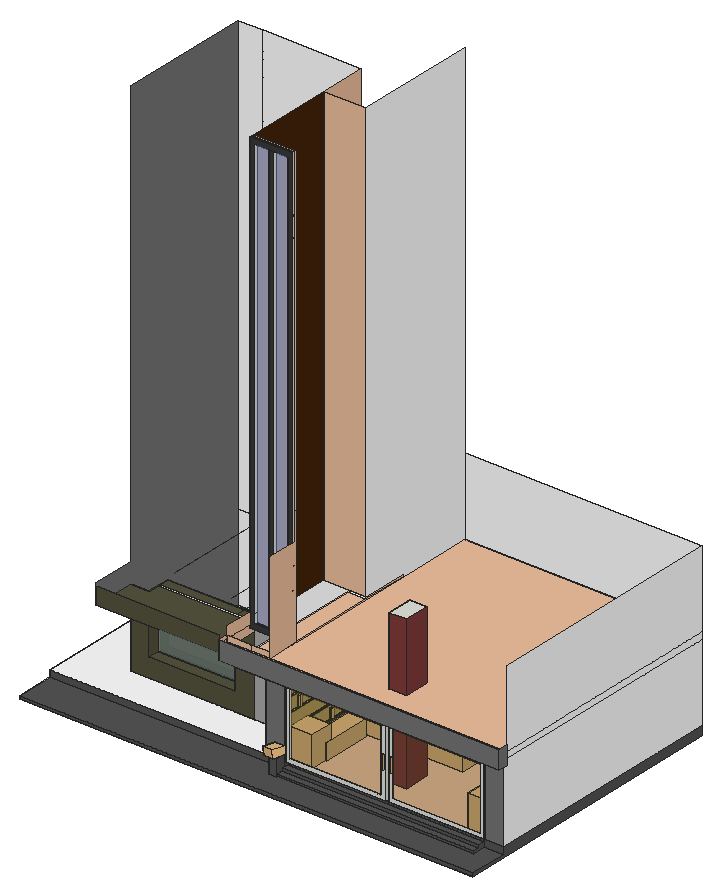
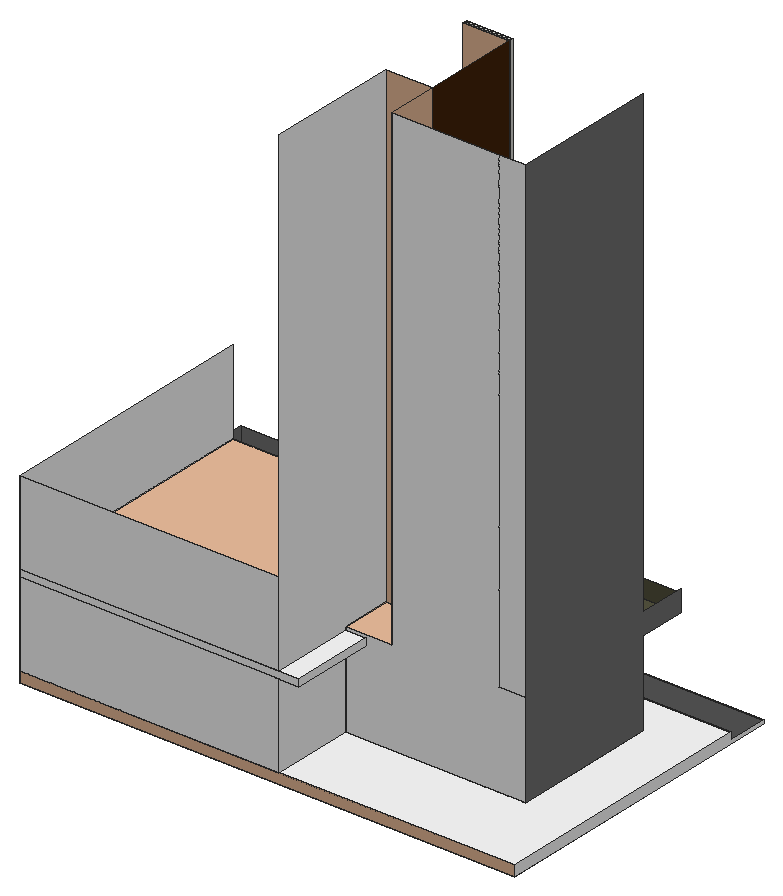
# SketchUp Ruby script. Lengths in inches.
U = 1.inch
M = Sketchup.active_model
def pt(a) = Geom::Point3d.new(a.map { |v| v * U })
def face(e, loops, mat)
  f = e.add_face(loops[0].map { |a| pt(a) })
  loops[1..].each { |l| e.add_face(l.map { |a| pt(a) }).erase! }
  f.material = f.back_material = mat if mat
  f
end
# faces: each face lists its corners as indices into pts; further lists are holes
def faces(e, pts, list, mat = nil) = list.each { |f| face(e, (f[0].is_a?(Array) ? f : [f]).map { |l| l.map { |i| pts[i] } }, mat) }
# xy, xz, yz: faces in a plane at the given z, y or x. An outline is a flat list of corners, or four numbers for a rectangle; further outlines are holes
def ring(l) = l.size == 4 ? [[l[0], l[1]], [l[2], l[1]], [l[2], l[3]], [l[0], l[3]]] : l.each_slice(2).to_a
def flat(e, list, mat, &to3) = list.each { |f| face(e, (f[0].is_a?(Array) ? f : [f]).map { |l| ring(l).map { |u, v| to3.(u, v) } }, mat) }
def xy(e, z, list, mat = nil) = flat(e, list, mat) { |x, y| [x, y, z] }
def xz(e, y, list, mat = nil) = flat(e, list, mat) { |x, z| [x, y, z] }
def yz(e, x, list, mat = nil) = flat(e, list, mat) { |y, z| [x, y, z] }
def lines(e, pts, list) = list.each { |a, b| e.add_line(pt(pts[a]), pt(pts[b])) }
# prism: a flat outline (further loops are holes) pulled along v
def prism(e, loops, v, mat = nil)
  f = face(e, loops, mat); d = Geom::Vector3d.new(v.map { |x| x * U })
  f.pushpull(f.normal.samedirection?(d) ? d.length : -d.length)
end
def box(e, o, s, mat = nil) = prism(e, [[o, [o[0] + s[0], o[1], o[2]], [o[0] + s[0], o[1] + s[1], o[2]], [o[0], o[1] + s[1], o[2]]]], [0, 0, s[2]], mat)
def at(x, y, z, deg = 0) = Geom::Transformation.translation(pt([x, y, z])) * Geom::Transformation.rotation(ORIGIN, Z_AXIS, deg.degrees)
def axes(o, x, y, z) = Geom::Transformation.new([*x, 0, *y, 0, *z, 0, *pt(o).to_a, 1])
def part(name) = M.definitions.add(name)
# library, detail: a bought-in or finely detailed component or shape, given as its bounding box
def library(name, o, s) = part(name).tap { |d| box(d.entities, o, s) }
def detail(e, o, s) = box(e.add_group.entities, o, s)
def put(e, d, t, mat = nil) = e.add_instance(d, t).tap { |i| i.material = mat if mat }
def group(e, t, mat = nil) = e.add_group.tap { |g| g.transformation = t; g.material = mat if mat }.entities
root = M.entities
M.materials.add("Generic").color = [68, 36, 11]
M.materials.add("Generic\#1").color = [84, 84, 84]
M.materials.add("Generic\#11").color = [129, 59, 59]
M.materials.add("Generic\#13").color = [239, 192, 158]
M.materials.add("Generic\#2").color = [84, 83, 62]
M.materials.add("Generic\#3").color = [117, 117, 117]
M.materials.add("Material__2").color = [190, 136, 85]
M.materials.add("Material__3").color = [51, 42, 44]
M.materials.add("Material__4").color = [119, 136, 107]
M.materials.add("[Color M00]").color = [255, 255, 255]
M.materials.add("[Color M03]").color = [170, 170, 170]
M.materials.add("[Color M07]").color = [58, 58, 58]
M.materials.add("[Mirror 02]").color = [230, 230, 157]
M.materials.add("[Translucent Glass Blue]").color = [100, 149, 237]
M.materials["[Translucent Glass Blue]"].alpha = 0.5
M.materials.add("[Translucent Glass Corrugated]").color = [177, 158, 60]
M.materials["[Translucent Glass Corrugated]"].alpha = 0.56
M.materials.add("[Translucent Glass Corrugated]1").color = [106, 119, 109]
M.materials["[Translucent Glass Corrugated]1"].alpha = 0.8
M.materials.add("[Translucent Glass Dark Green]").color = [86, 83, 28]
M.materials["[Translucent Glass Dark Green]"].alpha = 0.11
c1 = library("Plant+2 (1)",[-9.13,-9.52,0],[51.76,51.77,66.88])
c2 = library("cafe+table",[12.29,13.08,0],[75.61,73.69,46.46])
c3 = library("Group\#1",[0,0,0],[33.82,92.24,30.24])
c4 = part("Group\#7")
detail(c4.entities,[0,0,0],[1.625,2.25,24.9375])
c5 = library("\#2",[-119.83,-119.83,113.8],[239.66,239.66,17.4])
c6 = library("\#4",[-204.92,-212.35,-236.71],[424.28,257.5,472.53])
c7 = part("\#3")
put(c7.entities,c6,axes([-0.37,309.72,0],[1.36765,0,0],[0,1.36765,0],[0,0,1.36765]),"Material__4")
c8 = library("\#1",[-174.07,-174.07,0],[348.14,348.14,140])
c9 = part("9")
put(c9.entities,c5,at(-19.94,-24.66,0),"Material__3")
put(c9.entities,c7,axes([17.67,-32.6,40.29],[0.29694,0.9549,0],[-0.21403,0.06656,0.97456],[0.9306,-0.28939,0.22414]))
put(c9.entities,c8,at(-19.94,-24.66,0),"Material__2")
c10 = library("Wall Lamp 298 005",[-4.37,-9,-20.45],[8.74,9.125,40.9])
c11 = library("Untitled (6)",[-101.41,0,-4.6],[35.6,35.6,49.16])
c12 = library("Tlon Light 450 Ceiling 152 006",[-8.86,-8.86,-3.78],[17.72,17.72,3.56])
xy(root,-17.875,[[0,0,0,534.3125,848,534.3125,848,0,770.53,0,770.53,62.875,477.72,62.875,477.72,0],[477.72,0,770.53,62.875]],"Generic\#13")
xy(root,-12.4375,[[0,0,848,0,848,70.375,812,70.375,812,46.5,444.05,46.5,444.05,44.57,430.61,44.57,430.61,61.26,444.05,61.26,444.05,70.375,0,70.375]],"Generic\#1")
xy(root,-7.625,[[444.05,46.5,812,56.875]],"Generic\#1")
xy(root,-3.1875,[[444.05,56.875,812,70.375]],"Generic\#1")
xy(root,0,[[596.32,118.1875,628.39,166.25]])
xy(root,0,[[404,70.375,440,70.375,440,515.9375,812,515.9375,812,70.375,848,70.375,848,534.3125,404,534.3125],[440,70.375,442,78.3125],[442,70.375,810,514.9375],[810,70.375,812,78.3125],[440,78.3125,442,514.9375],
  [810,78.3125,812,514.9375],[94.0625,140.75,404,304.75],[94.0625,304.75,404,391.6875],[440,514.9375,812,515.9375],[440,514.9375,812,515.9375]],"Generic\#13")
xy(root,0,[[0,70.375,404,70.375,404,140.75,94.0625,140.75,94.0625,391.6875,404,391.6875,404,534.3125,0,534.3125]],"[Color M00]")
xy(root,17.3125,[[430.61,44.57,444.05,61.26]],"Generic\#1")
xy(root,23.6875,[[440,78.3125,442,514.9375],[810,78.3125,812,514.9375],[440,514.9375,812,515.9375]],"Generic\#13")
xy(root,26.6875,[[440,78.3125,442,514.9375],[810,78.3125,812,514.9375],[440,514.9375,812,515.9375]],"Generic\#13")
xy(root,35.01,[[129.07,140.75,289.24,184.8125]],"Generic\#2")
xy(root,50.375,[[440,78.3125,442,514.9375],[810,78.3125,812,514.9375],[440,514.9375,812,515.9375]],"Generic\#13")
xy(root,53.375,[[440,78.3125,442,514.9375],[810,78.3125,812,514.9375],[440,514.9375,812,515.9375]],"Generic\#13")
xy(root,77.0625,[[440,78.3125,442,514.9375],[810,78.3125,812,514.9375],[440,514.9375,812,515.9375]],"Generic\#13")
xy(root,80.0625,[[440,78.3125,442,514.9375],[810,78.3125,812,514.9375],[440,514.9375,812,515.9375]],"Generic\#13")
xy(root,103.75,[[440,78.3125,442,514.9375],[810,78.3125,812,514.9375],[440,514.9375,812,515.9375]],"Generic\#13")
xy(root,106.75,[[440,78.3125,442,514.9375],[810,78.3125,812,514.9375],[440,514.9375,812,515.9375]],"Generic\#13")
xy(root,133.4375,[[404,70.375,440,78.3125],[440,70.375,810,78.3125],[810,70.375,812,78.3125],[812,70.375,848,78.3125],[440,78.3125,442,514.9375],
  [442,78.3125,810,514.9375],[810,78.3125,812,514.9375],[440,514.9375,812,515.9375]],"Generic\#13")
xy(root,133.4375,[[324.25,60.4375,848,70.375],[324.25,70.375,404,78.3125]],"Generic\#3")
xy(root,144,[[369.1875,78.3125,404,534.3125],[404,78.3125,848,534.3125]],"Generic\#13")
xy(root,145.5625,[[94.0625,60.4375,94.0625,140.75,129.07,140.75,129.07,184.8125,289.24,184.8125,289.24,140.75,324.25,140.75,324.25,60.4375]],"Generic\#2")
xy(root,156.625,[[369.1875,78.3125,404,140.75],[404,78.3125,848,534.3125],[369.1875,140.75,404,304.75]],"Generic\#13")
xy(root,156.625,[[369.1875,304.75,404,534.3125]],"[Color M00]")
xy(root,161.19,[[324.25,304.75,404,391.6875]],"Generic\#13")
xy(root,284,[[596.32,118.1875,628.39,166.25]])
xz(root,0,[[0,-17.875,848,-12.4375]],"Generic\#1")
xz(root,44.57,[[430.61,-12.4375,444.05,17.3125]],"Generic\#1")
xz(root,46.5,[[444.05,-12.4375,812,-7.625]],"Generic\#1")
xz(root,56.875,[[444.05,-7.625,812,-3.1875]],"Generic\#1")
xz(root,60.4375,[[94.0625,145.5625,324.25,176.75]],"Generic\#2")
xz(root,60.4375,[[324.25,133.4375,848,168.25]],"Generic\#3")
xz(root,61.26,[[430.61,-12.4375,444.05,17.3125]],"Generic\#1")
xz(root,70.375,[[0,-12.4375,444.05,-12.4375,444.05,-3.1875,812,-3.1875,812,-12.4375,848,-12.4375,848,0,0,0]],"Generic\#1")
xz(root,70.375,[[404,0,440,133.4375],[812,0,848,133.4375]],"Generic\#3")
xz(root,78.3125,[[440,0,442,23.6875],[810,0,812,23.6875],[440,26.6875,442,50.375],[810,26.6875,812,50.375],[440,53.375,442,77.0625],
  [810,53.375,812,77.0625],[440,80.0625,442,103.75],[810,80.0625,812,103.75],[440,106.75,442,133.4375],[810,106.75,812,133.4375],
  [324.25,133.4375,404,144],[404,133.4375,848,144],[324.25,144,369.1875,156.625],[369.1875,144,848,156.625],[324.25,156.625,369.1875,168.25],
  [369.1875,156.625,404,168.25]],"Generic\#13")
xz(root,118.1875,[[596.32,0,628.39,284]],"Generic\#11")
xz(root,140.75,[[324.25,156.625,404,979.625]],"Generic\#13")
xz(root,140.75,[[94.0625,0,324.25,0,324.25,145.5625,289.24,145.5625,289.24,35.01,129.07,35.01,129.07,145.5625,94.0625,145.5625]],"Generic\#2")
xz(root,140.75,[[324.25,0,404,156.625]],"[Color M03]")
xz(root,166.25,[[596.32,0,628.39,284]])
xz(root,184.8125,[[129.07,35.01,289.24,145.5625]])
xz(root,304.75,[[324.25,161.19,404,979.625]],"Generic\#13")
xz(root,391.6875,[[94.0625,0,94.0625,161.19,141.125,161.19,141.125,979.625,324.25,979.625,324.25,161.19,404,161.19,404,0],[94.0625,161.19,141.125,979.625]],"[Color M00]")
xz(root,514.9375,[[440,0,442,23.6875],[810,0,812,23.6875],[440,26.6875,442,50.375],[810,26.6875,812,50.375],[440,53.375,442,77.0625],
  [810,53.375,812,77.0625],[440,80.0625,442,103.75],[810,80.0625,812,103.75],[440,106.75,442,133.4375],[810,106.75,812,133.4375]],"Generic\#13")
xz(root,514.9375,[[442,0,810,23.6875],[442,26.6875,810,50.375],[442,53.375,810,77.0625],[442,80.0625,810,103.75],[442,106.75,810,133.4375]],"[Translucent Glass Corrugated]")
xz(root,515.9375,[[440,0,812,23.6875],[440,26.6875,812,50.375],[440,53.375,812,77.0625],[440,80.0625,812,103.75],[440,106.75,812,133.4375]],"Generic\#13")
xz(root,515.9375,[[440,23.6875,812,26.6875],[440,50.375,812,53.375],[440,77.0625,812,80.0625],[440,103.75,812,106.75]],"[Mirror 02]")
xz(root,534.3125,[[0,-17.875,848,0]],"Generic\#13")
xz(root,534.3125,[[404,0,848,144],[369.1875,144,848,156.625],[404,156.625,848,300.625]],"[Color M00]")
yz(root,0,[[0,-17.875,0,-12.4375,70.375,-12.4375,70.375,0,534.3125,0,534.3125,-17.875]],"[Color M00]")
yz(root,94.0625,[[140.75,0,140.75,145.5625,60.4375,145.5625,60.4375,182.75,140.75,182.75,140.75,979.625,391.6875,979.625,391.6875,0]],"Generic\#3")
yz(root,129.07,[[140.75,35.01,184.8125,145.5625]],"Generic\#2")
yz(root,289.24,[[140.75,35.01,184.8125,145.5625]],"Generic\#2")
yz(root,324.25,[[140.75,161.19,304.75,979.625]],"Generic")
yz(root,324.25,[[60.4375,145.5625,78.3125,161.19],[78.3125,145.5625,140.75,161.19],[60.4375,161.19,78.3125,168.25],[78.3125,161.19,140.75,182.75],[304.75,161.19,391.6875,979.625]],"Generic\#13")
yz(root,324.25,[[60.4375,133.4375,70.375,145.5625],[70.375,133.4375,78.3125,145.5625]],"Generic\#3")
yz(root,369.1875,[[78.3125,144,534.3125,156.625]],"[Color M00]")
yz(root,404,[[70.375,0,70.375,133.4375,78.3125,133.4375,78.3125,144,140.75,144,140.75,0],[140.75,0,304.75,144],[304.75,0,391.6875,144],[140.75,144,304.75,156.625],[304.75,144,391.6875,156.625],
  [78.3125,156.625,78.3125,326.375,136.9375,326.375,136.9375,377.0625,140.75,377.0625,140.75,156.625],[304.75,156.625,391.6875,161.19]],"Generic\#13")
yz(root,404,[[391.6875,0,534.3125,144],[391.6875,156.625,391.6875,161.19,304.75,161.19,304.75,979.625,534.3125,979.625,534.3125,156.625]],"[Color M00]")
yz(root,430.61,[[44.57,-12.4375,61.26,17.3125]],"Generic\#1")
yz(root,440,[[70.375,0,78.3125,23.6875],[78.3125,0,514.9375,23.6875],[514.9375,0,515.9375,23.6875],[70.375,26.6875,78.3125,50.375],[78.3125,26.6875,514.9375,50.375],
  [514.9375,26.6875,515.9375,50.375],[70.375,53.375,78.3125,77.0625],[78.3125,53.375,514.9375,77.0625],[514.9375,53.375,515.9375,77.0625],[70.375,80.0625,78.3125,103.75],
  [78.3125,80.0625,514.9375,103.75],[514.9375,80.0625,515.9375,103.75],[70.375,106.75,78.3125,133.4375],[78.3125,106.75,514.9375,133.4375],[514.9375,106.75,515.9375,133.4375]],"Generic\#13")
yz(root,440,[[70.375,23.6875,515.9375,26.6875],[70.375,50.375,515.9375,53.375],[70.375,77.0625,515.9375,80.0625],[70.375,103.75,515.9375,106.75]],"[Mirror 02]")
yz(root,442,[[78.3125,0,514.9375,23.6875],[78.3125,26.6875,514.9375,50.375],[78.3125,53.375,514.9375,77.0625],[78.3125,80.0625,514.9375,103.75],[78.3125,106.75,514.9375,133.4375]],"[Translucent Glass Corrugated]")
yz(root,444.05,[[44.57,-12.4375,46.5,-12.4375,46.5,-7.625,56.875,-7.625,56.875,-3.1875,61.26,-3.1875,61.26,17.3125,44.57,17.3125],[46.5,-12.4375,61.26,-12.4375,61.26,-3.1875,56.875,-3.1875,56.875,-7.625,46.5,-7.625],[61.26,-12.4375,70.375,-3.1875]],"Generic\#1")
yz(root,596.32,[[118.1875,0,166.25,284]],"Generic\#11")
yz(root,628.39,[[118.1875,0,166.25,284]],"Generic\#11")
yz(root,810,[[78.3125,0,514.9375,23.6875],[78.3125,26.6875,514.9375,50.375],[78.3125,53.375,514.9375,77.0625],[78.3125,80.0625,514.9375,103.75],[78.3125,106.75,514.9375,133.4375]],"[Translucent Glass Corrugated]")
yz(root,812,[[46.5,-12.4375,70.375,-12.4375,70.375,-3.1875,56.875,-3.1875,56.875,-7.625,46.5,-7.625]],"Generic\#1")
yz(root,812,[[70.375,0,78.3125,23.6875],[78.3125,0,514.9375,23.6875],[514.9375,0,515.9375,23.6875],[70.375,26.6875,78.3125,50.375],[78.3125,26.6875,514.9375,50.375],
  [514.9375,26.6875,515.9375,50.375],[70.375,53.375,78.3125,77.0625],[78.3125,53.375,514.9375,77.0625],[514.9375,53.375,515.9375,77.0625],[70.375,80.0625,78.3125,103.75],
  [78.3125,80.0625,514.9375,103.75],[514.9375,80.0625,515.9375,103.75],[70.375,106.75,78.3125,133.4375],[78.3125,106.75,514.9375,133.4375],[514.9375,106.75,515.9375,133.4375]],"Generic\#13")
yz(root,812,[[70.375,23.6875,515.9375,26.6875],[70.375,50.375,515.9375,53.375],[70.375,77.0625,515.9375,80.0625],[70.375,103.75,515.9375,106.75]],"[Mirror 02]")
yz(root,848,[[0,-17.875,534.3125,-17.875,534.3125,0,70.375,0,70.375,-12.4375,0,-12.4375]],"Generic\#1")
yz(root,848,[[60.4375,133.4375,78.3125,168.25]],"Generic\#3")
yz(root,848,[[70.375,0,534.3125,0,534.3125,144,78.3125,144,78.3125,133.4375,70.375,133.4375],[78.3125,144,534.3125,156.625],[78.3125,156.625,534.3125,300.625]],"[Color M00]")
p = [[248,304.75,156.625],[248,184.8125,156.625],[141.125,184.8125,161.19],[141.125,391.6875,161.19],[289.24,184.8125,161.19],[289.24,184.8125,145.5625],
  [289.24,140.75,161.19]]
lines(root,p,[[0,1],[2,3],[4,5],[4,6]])
put(root,c1,axes([447.56,86.96,0],[0.8385,0,0],[0,0.8385,0],[0,0,0.8385]))
put(root,c1,axes([782.91,87.7,0],[0.9165,0,0],[0,0.9165,0],[0,0,0.9165]))
put(root,c2,at(442,404.72,0))
put(root,c2,at(573.0625,404.72,0))
put(root,c2,at(696.0625,404.72,0))
put(root,c2,at(696.0625,292.03,0))
put(root,c2,at(442,292.03,0))
put(root,c2,at(573.0625,292.03,0))
put(root,c2,at(696.0625,195.28,0))
put(root,c2,at(442,195.28,0))
put(root,c2,at(573.0625,195.28,0))
put(root,c3,at(486.49,201.24,0,180))
g1 = group(root,at(442,68.125,0))
xy(g1,0,[[0,1.625,2,8.25],[2,1.625,186,8.25],[192,2.25,370,8.25],[370,2.25,372,8.25]])
xy(g1,8,[[8,1.625,178,2.25]])
xy(g1,125.4375,[[8,1.625,178,2.25]])
xy(g1,133.4375,[[0,1.625,186,8.25],[192,2.25,370,8.25],[370,2.25,372,8.25]])
xz(g1,1.625,[[[0,0,186,133.4375],[8,8,178,125.4375],[182.1,75.14,181.89,75.16,181.6875,75.24,181.52,75.375,181.39,75.54,181.3125,75.74,181.28,75.95,181.3125,76.16,181.39,76.35,181.52,76.52,181.6875,76.65,181.89,76.73,182.1,76.76,182.31,76.73,182.5,76.65,182.67,76.52,182.8,76.35,182.88,76.16,182.91,75.95,182.88,75.74,182.8,75.54,182.67,75.375,182.5,75.24,182.31,75.16],[182.1,51.82,181.89,51.85,181.6875,51.93,181.52,52.0625,181.39,52.23,181.3125,52.43,181.28,52.64,181.3125,52.85,181.39,53.04,181.52,53.21,181.6875,53.34,181.89,53.42,182.1,53.45,182.31,53.42,182.5,53.34,182.67,53.21,182.8,53.04,182.88,52.85,182.91,52.64,182.88,52.43,182.8,52.23,182.67,52.0625,182.5,51.93,182.31,51.85]]])
xz(g1,2.25,[[[192,0,372,133.4375],[200,8,364,125.4375]],[182.1,75.14,181.89,75.16,181.6875,75.24,181.52,75.375,181.39,75.54,181.3125,75.74,181.28,75.95,181.3125,76.16,181.39,76.35,181.52,76.52,181.6875,76.65,181.89,76.73,182.1,76.76,182.31,76.73,182.5,76.65,182.67,76.52,182.8,76.35,182.88,76.16,182.91,75.95,182.88,75.74,182.8,75.54,182.67,75.375,182.5,75.24,182.31,75.16]])
xz(g1,2.25,[[8,8,178,125.4375],[200,8,364,125.4375]],"[Translucent Glass Dark Green]")
xz(g1,8.25,[[0,0,186,133.4375],[192,0,372,133.4375]],"[Translucent Glass Dark Green]")
yz(g1,0,[[1.625,0,8.25,133.4375]])
yz(g1,8,[[1.625,8,2.25,125.4375]])
yz(g1,178,[[1.625,8,2.25,125.4375]])
yz(g1,186,[[1.625,0,8.25,133.4375]])
yz(g1,192,[[2.25,0,8.25,133.4375]])
yz(g1,372,[[2.25,0,8.25,133.4375]])
p = [[182.1,2.25,51.82],[181.89,2.25,51.85],[181.89,1.625,51.85],[182.1,1.625,51.82],[182.31,2.25,51.85],[182.31,1.625,51.85],
  [181.6875,2.25,51.93],[181.52,2.25,52.0625],[181.52,1.625,52.0625],[181.6875,1.625,51.93],[182.5,2.25,51.93],[182.5,1.625,51.93],
  [182.67,2.25,52.0625],[182.67,1.625,52.0625],[181.39,2.25,52.23],[181.39,1.625,52.23],[182.8,2.25,52.23],[182.8,1.625,52.23],
  [181.3125,2.25,52.43],[181.3125,1.625,52.43],[182.88,2.25,52.43],[182.88,1.625,52.43],[181.28,2.25,52.64],[181.28,1.625,52.64],
  [182.91,2.25,52.64],[182.91,1.625,52.64],[181.3125,2.25,52.85],[181.3125,1.625,52.85],[182.88,2.25,52.85],[182.88,1.625,52.85],
  [181.39,2.25,53.04],[181.39,1.625,53.04],[182.8,2.25,53.04],[182.8,1.625,53.04],[181.52,2.25,53.21],[181.52,1.625,53.21],
  [182.67,2.25,53.21],[182.67,1.625,53.21],[181.6875,2.25,53.34],[181.6875,1.625,53.34],[182.5,2.25,53.34],[182.5,1.625,53.34],
  [181.89,2.25,53.42],[181.89,1.625,53.42],[182.31,2.25,53.42],[182.31,1.625,53.42],[182.1,2.25,53.45],[182.1,1.625,53.45],
  [182.1,2.25,75.14],[181.89,2.25,75.16],[181.89,1.625,75.16],[182.1,1.625,75.14],[182.31,2.25,75.16],[182.31,1.625,75.16],
  [181.6875,2.25,75.24],[181.52,2.25,75.375],[181.52,1.625,75.375],[181.6875,1.625,75.24],[182.5,2.25,75.24],[182.5,1.625,75.24],
  [182.67,2.25,75.375],[182.67,1.625,75.375],[181.39,2.25,75.54],[181.39,1.625,75.54],[182.8,2.25,75.54],[182.8,1.625,75.54],
  [181.3125,2.25,75.74],[181.3125,1.625,75.74],[182.88,2.25,75.74],[182.88,1.625,75.74],[181.28,2.25,75.95],[181.28,1.625,75.95],
  [182.91,2.25,75.95],[182.91,1.625,75.95],[181.3125,2.25,76.16],[181.3125,1.625,76.16],[182.88,2.25,76.16],[182.88,1.625,76.16],
  [181.39,2.25,76.35],[181.39,1.625,76.35],[182.8,2.25,76.35],[182.8,1.625,76.35],[181.52,2.25,76.52],[181.52,1.625,76.52],
  [182.67,2.25,76.52],[182.67,1.625,76.52],[181.6875,2.25,76.65],[181.6875,1.625,76.65],[182.5,2.25,76.65],[182.5,1.625,76.65],
  [181.89,2.25,76.73],[181.89,1.625,76.73],[182.1,2.25,76.76],[182.1,1.625,76.76],[182.31,2.25,76.73],[182.31,1.625,76.73],
  [186,8.25,0],[192,8.25,0],[182.1,2.25,75.95],[182.1,0.8125,75.95],[182.1,0.8125,52.64],[182.1,2.25,52.64]]
faces(g1,p,[[0,1,2,3],[4,0,3,5],[6,7,8,9],[1,6,9,2],[10,4,5,11],[12,10,11,13],[7,14,15,8],[16,12,13,17],
  [14,18,19,15],[20,16,17,21],[18,22,23,19],[24,20,21,25],[22,26,27,23],[28,24,25,29],[26,30,31,27],[32,28,29,33],
  [30,34,35,31],[36,32,33,37],[34,38,39,35],[40,36,37,41],[38,42,43,39],[44,40,41,45],[42,46,47,43],[46,44,45,47],
  [48,49,50,51],[52,48,51,53],[54,55,56,57],[49,54,57,50],[58,52,53,59],[60,58,59,61],[55,62,63,56],[64,60,61,65],
  [62,66,67,63],[68,64,65,69],[66,70,71,67],[72,68,69,73],[70,74,75,71],[76,72,73,77],[74,78,79,75],[80,76,77,81],
  [78,82,83,79],[84,80,81,85],[82,86,87,83],[88,84,85,89],[86,90,91,87],[90,92,93,91],[92,94,95,93],[94,88,89,95]])
lines(g1,p,[[96,97],[98,99],[99,100],[100,101]])
put(g1,c4,at(195.35,0,51.82))
put(g1,c4,at(181.28,0,51.82))
put(root,c3,at(763.72,106,0))
put(root,c9,axes([436.23,50.24,17.83],[0.03845,0,0],[0,0.03845,0],[0,0,0.03845]))
put(root,c10,axes([443.33,98.76,38.57],[0,0.4284,0],[-0.4284,0,0],[0,0,0.4284]))
put(root,c10,axes([443.33,172.51,38.57],[0,0.4284,0],[-0.4284,0,0],[0,0,0.4284]))
put(root,c10,axes([443.33,262.51,38.57],[0,0.4284,0],[-0.4284,0,0],[0,0,0.4284]))
put(root,c10,axes([443.33,338.82,38.57],[0,0.4284,0],[-0.4284,0,0],[0,0,0.4284]))
put(root,c10,axes([443.33,411.38,38.57],[0,0.4284,0],[-0.4284,0,0],[0,0,0.4284]))
put(root,c10,axes([443.33,494.32,38.57],[0,0.4284,0],[-0.4284,0,0],[0,0,0.4284]))
put(root,c10,axes([467.02,514.88,38.7],[0.4284,0,0],[0,0.4284,0],[0,0,0.4284]))
put(root,c10,axes([507.14,514.88,38.7],[0.4284,0,0],[0,0.4284,0],[0,0,0.4284]))
put(root,c10,axes([564.83,514.88,38.7],[0.4284,0,0],[0,0.4284,0],[0,0,0.4284]))
put(root,c10,axes([613.46,514.88,38.7],[0.4284,0,0],[0,0.4284,0],[0,0,0.4284]))
put(root,c10,axes([688.39,514.88,38.7],[0.4284,0,0],[0,0.4284,0],[0,0,0.4284]))
put(root,c10,axes([769.66,514.88,38.7],[0.4284,0,0],[0,0.4284,0],[0,0,0.4284]))
g2 = group(root,at(129.07,162.78,35.01))
xy(g2,0,[[0,0,160.18,3]])
xy(g2,110.56,[[0,0,160.18,3]])
xz(g2,0,[[0,0,160.18,110.56]],"[Translucent Glass Corrugated]1")
xz(g2,3,[[0,0,160.18,110.56]],"[Translucent Glass Corrugated]1")
yz(g2,0,[[0,0,3,110.56]])
yz(g2,160.18,[[0,0,3,92.3],[0,92.3,3,98.43],[0,98.43,3,110.56]])
put(root,c11,axes([600.6875,230.23,79.24],[0.79048,0,0],[0,0.5478,0],[0,0,1.21612]))
put(root,c11,axes([618.6875,381.42,79.24],[0.79048,0,0],[0,0.5478,0],[0,0,1.21612]))
put(root,c11,axes([779.3125,381.42,79.24],[0.79048,0,0],[0,0.5478,0],[0,0,1.21612]))
put(root,c11,axes([804.9375,230.23,79.24],[0.79048,0,0],[0,0.5478,0],[0,0,1.21612]))
put(root,c10,axes([467.02,514.88,91.7],[0.4284,0,0],[0,0.4284,0],[0,0,0.4284]))
put(root,c10,axes([510.08,514.88,91.7],[0.4284,0,0],[0,0.4284,0],[0,0,0.4284]))
put(root,c10,axes([561.71,514.88,91.7],[0.4284,0,0],[0,0.4284,0],[0,0,0.4284]))
put(root,c10,axes([617.14,514.88,91.7],[0.4284,0,0],[0,0.4284,0],[0,0,0.4284]))
put(root,c10,axes([689.14,514.88,91.7],[0.4284,0,0],[0,0.4284,0],[0,0,0.4284]))
put(root,c10,axes([775.21,514.88,91.7],[0.4284,0,0],[0,0.4284,0],[0,0,0.4284]))
put(root,c10,axes([443.33,98.76,92.19],[0,0.4284,0],[-0.4284,0,0],[0,0,0.4284]))
put(root,c10,axes([443.33,194.13,92.19],[0,0.4284,0],[-0.4284,0,0],[0,0,0.4284]))
put(root,c10,axes([443.33,269.76,92.19],[0,0.4284,0],[-0.4284,0,0],[0,0,0.4284]))
put(root,c10,axes([443.33,346.13,92.19],[0,0.4284,0],[-0.4284,0,0],[0,0,0.4284]))
put(root,c10,axes([443.33,429.95,92.19],[0,0.4284,0],[-0.4284,0,0],[0,0,0.4284]))
put(root,c12,axes([767.95,104.38,135.27],[0.64,0,0],[0,0.64,0],[0,0,0.64]))
put(root,c12,axes([767.95,169.44,135.27],[0.64,0,0],[0,0.64,0],[0,0,0.64]))
put(root,c12,axes([767.95,234.51,135.27],[0.64,0,0],[0,0.64,0],[0,0,0.64]))
put(root,c12,axes([767.95,299.57,135.27],[0.64,0,0],[0,0.64,0],[0,0,0.64]))
put(root,c12,axes([767.95,364.63,135.27],[0.64,0,0],[0,0.64,0],[0,0,0.64]))
put(root,c12,axes([767.95,429.69,135.27],[0.64,0,0],[0,0.64,0],[0,0,0.64]))
put(root,c12,axes([689.26,104.38,135.27],[0.64,0,0],[0,0.64,0],[0,0,0.64]))
put(root,c12,axes([689.26,234.51,135.27],[0.64,0,0],[0,0.64,0],[0,0,0.64]))
put(root,c12,axes([689.26,169.44,135.27],[0.64,0,0],[0,0.64,0],[0,0,0.64]))
put(root,c12,axes([689.26,299.57,135.27],[0.64,0,0],[0,0.64,0],[0,0,0.64]))
put(root,c12,axes([689.26,429.69,135.27],[0.64,0,0],[0,0.64,0],[0,0,0.64]))
put(root,c12,axes([689.26,364.63,135.27],[0.64,0,0],[0,0.64,0],[0,0,0.64]))
put(root,c12,axes([588.51,169.44,135.27],[0.64,0,0],[0,0.64,0],[0,0,0.64]))
put(root,c12,axes([588.51,429.69,135.27],[0.64,0,0],[0,0.64,0],[0,0,0.64]))
put(root,c12,axes([588.51,364.63,135.27],[0.64,0,0],[0,0.64,0],[0,0,0.64]))
put(root,c12,axes([588.51,299.57,135.27],[0.64,0,0],[0,0.64,0],[0,0,0.64]))
put(root,c12,axes([588.51,234.51,135.27],[0.64,0,0],[0,0.64,0],[0,0,0.64]))
put(root,c12,axes([588.51,104.38,135.27],[0.64,0,0],[0,0.64,0],[0,0,0.64]))
put(root,c12,axes([498.26,429.69,135.27],[0.64,0,0],[0,0.64,0],[0,0,0.64]))
put(root,c12,axes([498.26,364.63,135.27],[0.64,0,0],[0,0.64,0],[0,0,0.64]))
put(root,c12,axes([498.26,234.51,135.27],[0.64,0,0],[0,0.64,0],[0,0,0.64]))
put(root,c12,axes([498.26,169.44,135.27],[0.64,0,0],[0,0.64,0],[0,0,0.64]))
put(root,c12,axes([498.26,104.38,135.27],[0.64,0,0],[0,0.64,0],[0,0,0.64]))
put(root,c12,axes([498.26,299.57,135.27],[0.64,0,0],[0,0.64,0],[0,0,0.64]))
g3 = group(root,at(324.25,132.125,156.625))
xy(g3,0,[[0,0,44.9375,3.9375],[44.9375,0,79.75,3.9375]])
xy(g3,9.36,[[9.36,0,35.3125,3.9375],[35.3125,0,44.9375,3.9375],[44.9375,0,70.39,3.9375]])
xy(g3,813.64,[[9.36,0,35.3125,3.9375],[35.3125,0,44.9375,3.9375],[44.9375,0,70.39,3.9375]])
xy(g3,823,[[0,0,79.75,3.9375]])
xz(g3,0,[[[0,0,79.75,823],[9.36,9.36,70.39,813.64]],[35.3125,9.36,44.9375,813.64]],"[Color M07]")
xz(g3,3.9375,[[[0,0,79.75,823],[9.36,9.36,70.39,813.64]]])
xz(g3,3.9375,[[9.36,9.36,35.3125,813.64],[44.9375,9.36,70.39,813.64]],"[Translucent Glass Blue]")
yz(g3,0,[[0,0,3.9375,4.56],[0,4.56,3.9375,26.125],[0,26.125,3.9375,823]])
yz(g3,9.36,[[0,9.36,3.9375,26.125],[0,26.125,3.9375,813.64]])
yz(g3,35.3125,[[0,9.36,3.9375,26.125],[0,26.125,3.9375,813.64]])
yz(g3,44.9375,[[0,9.36,3.9375,26.125],[0,26.125,3.9375,813.64]])
yz(g3,70.39,[[0,9.36,3.9375,26.125],[0,26.125,3.9375,679],[0,679,3.9375,716.4375],[0,716.4375,3.9375,720.5625],[0,720.5625,3.9375,813.64]])
yz(g3,79.75,[[0,0,3.9375,679],[0,679,3.9375,716.4375],[0,716.4375,3.9375,720.5625],[0,720.5625,3.9375,823]])
